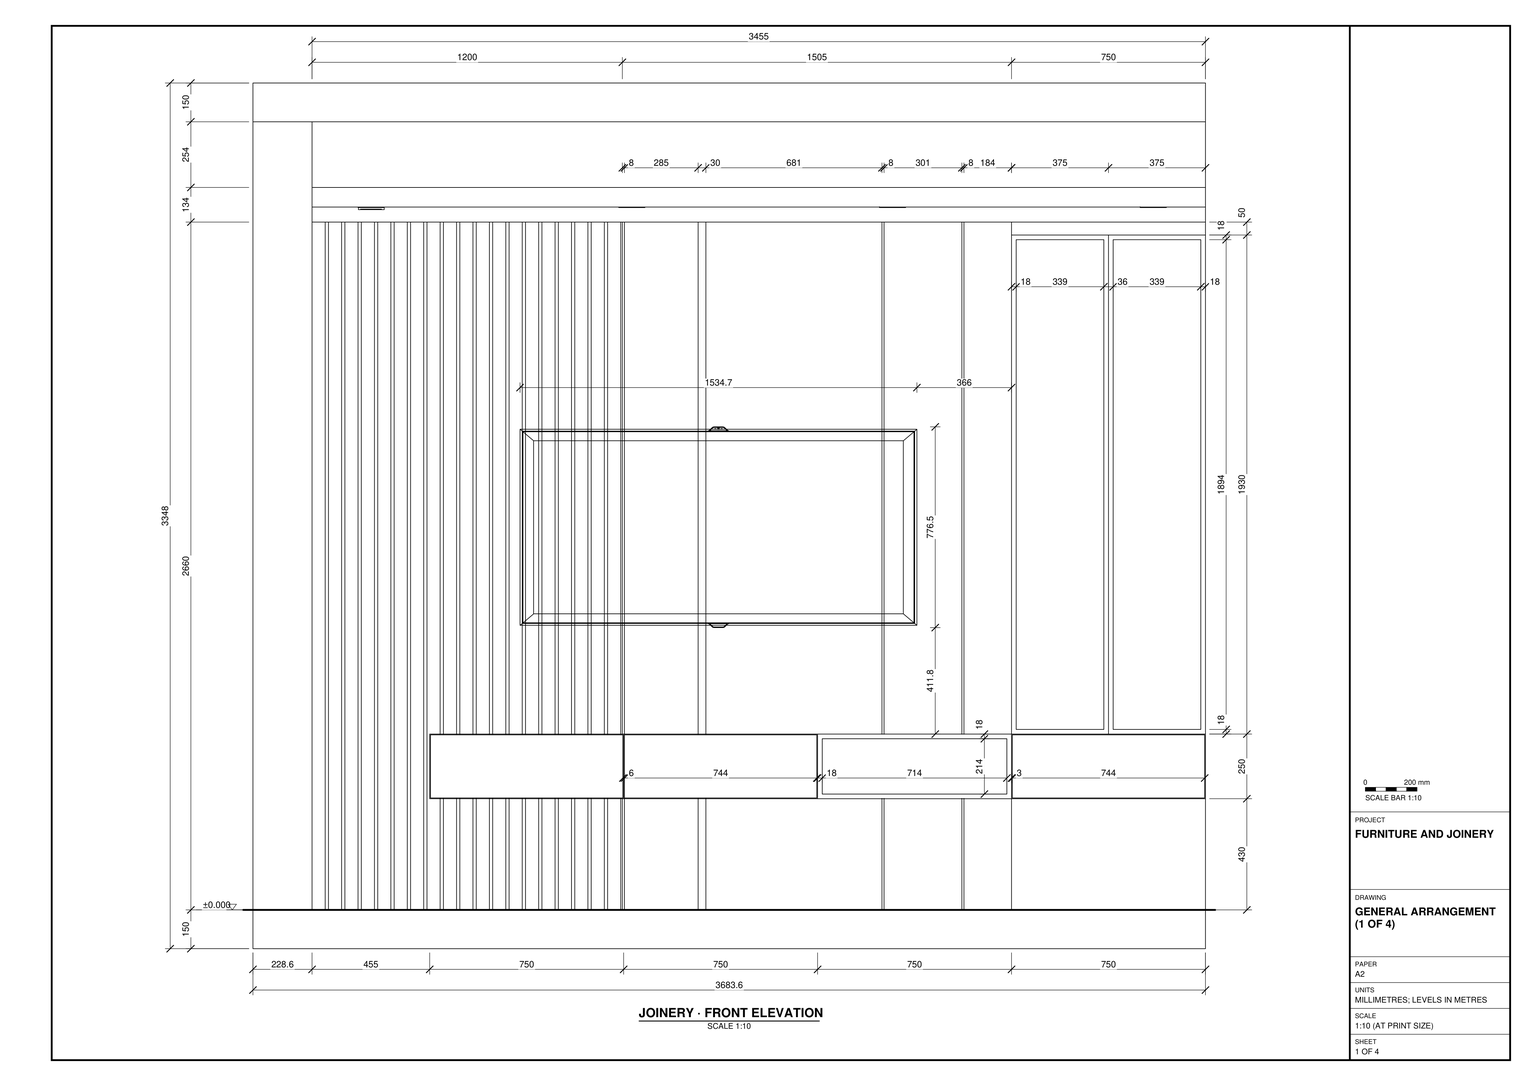
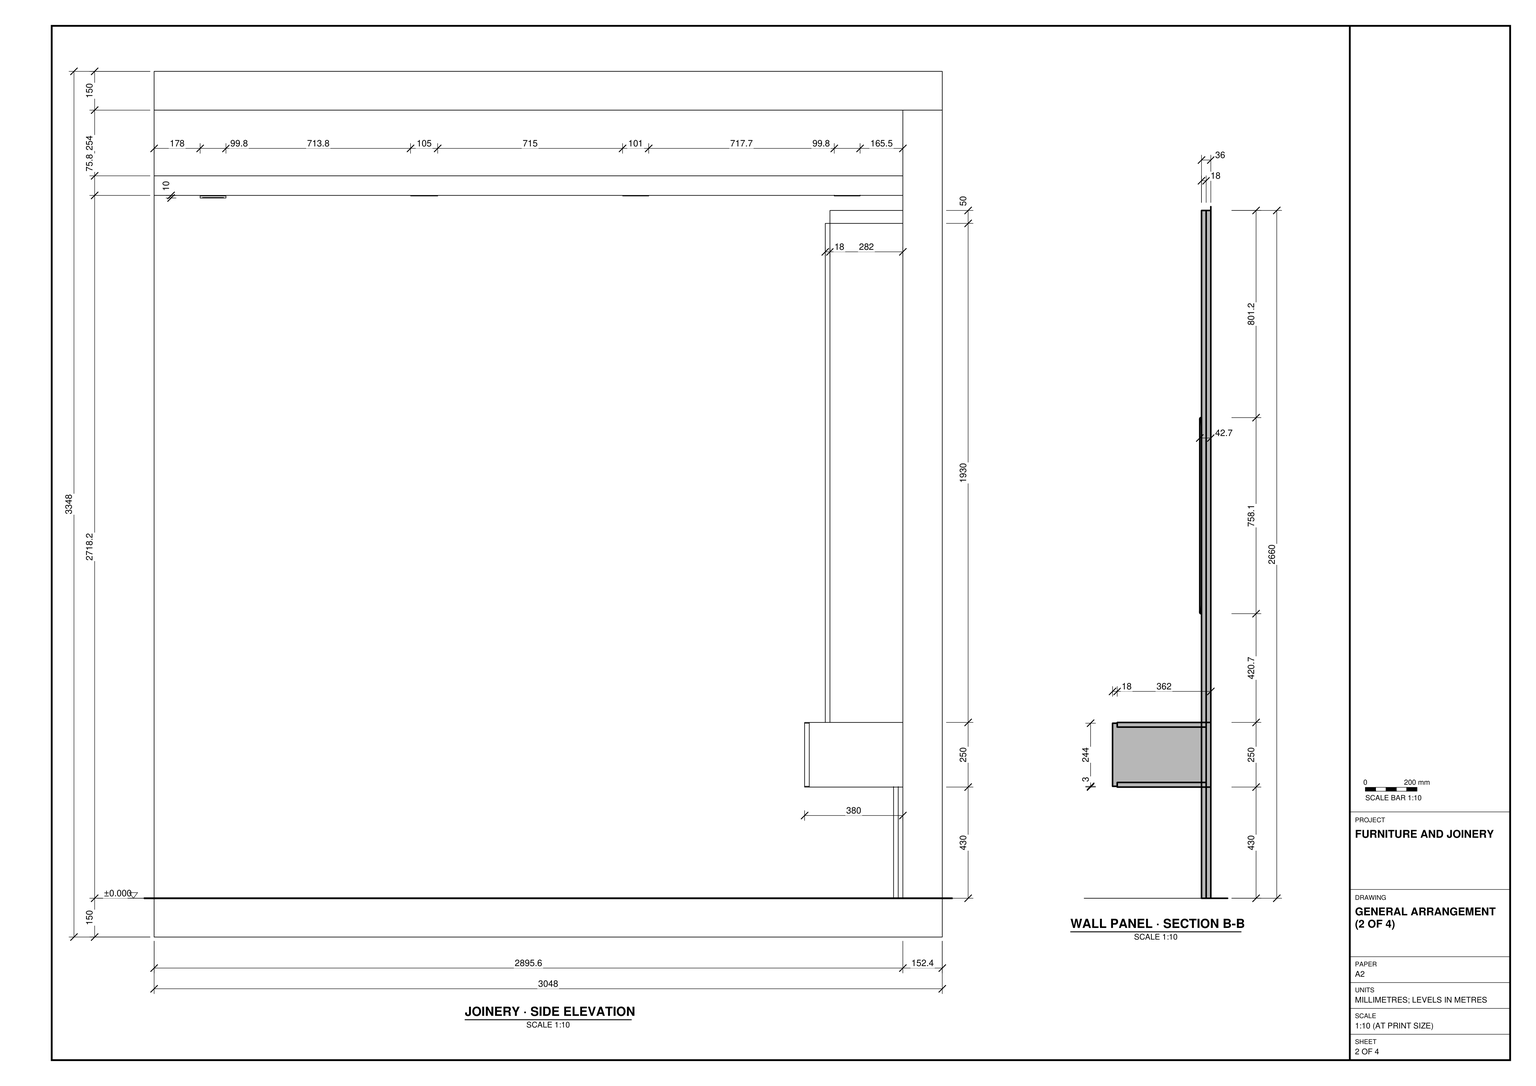
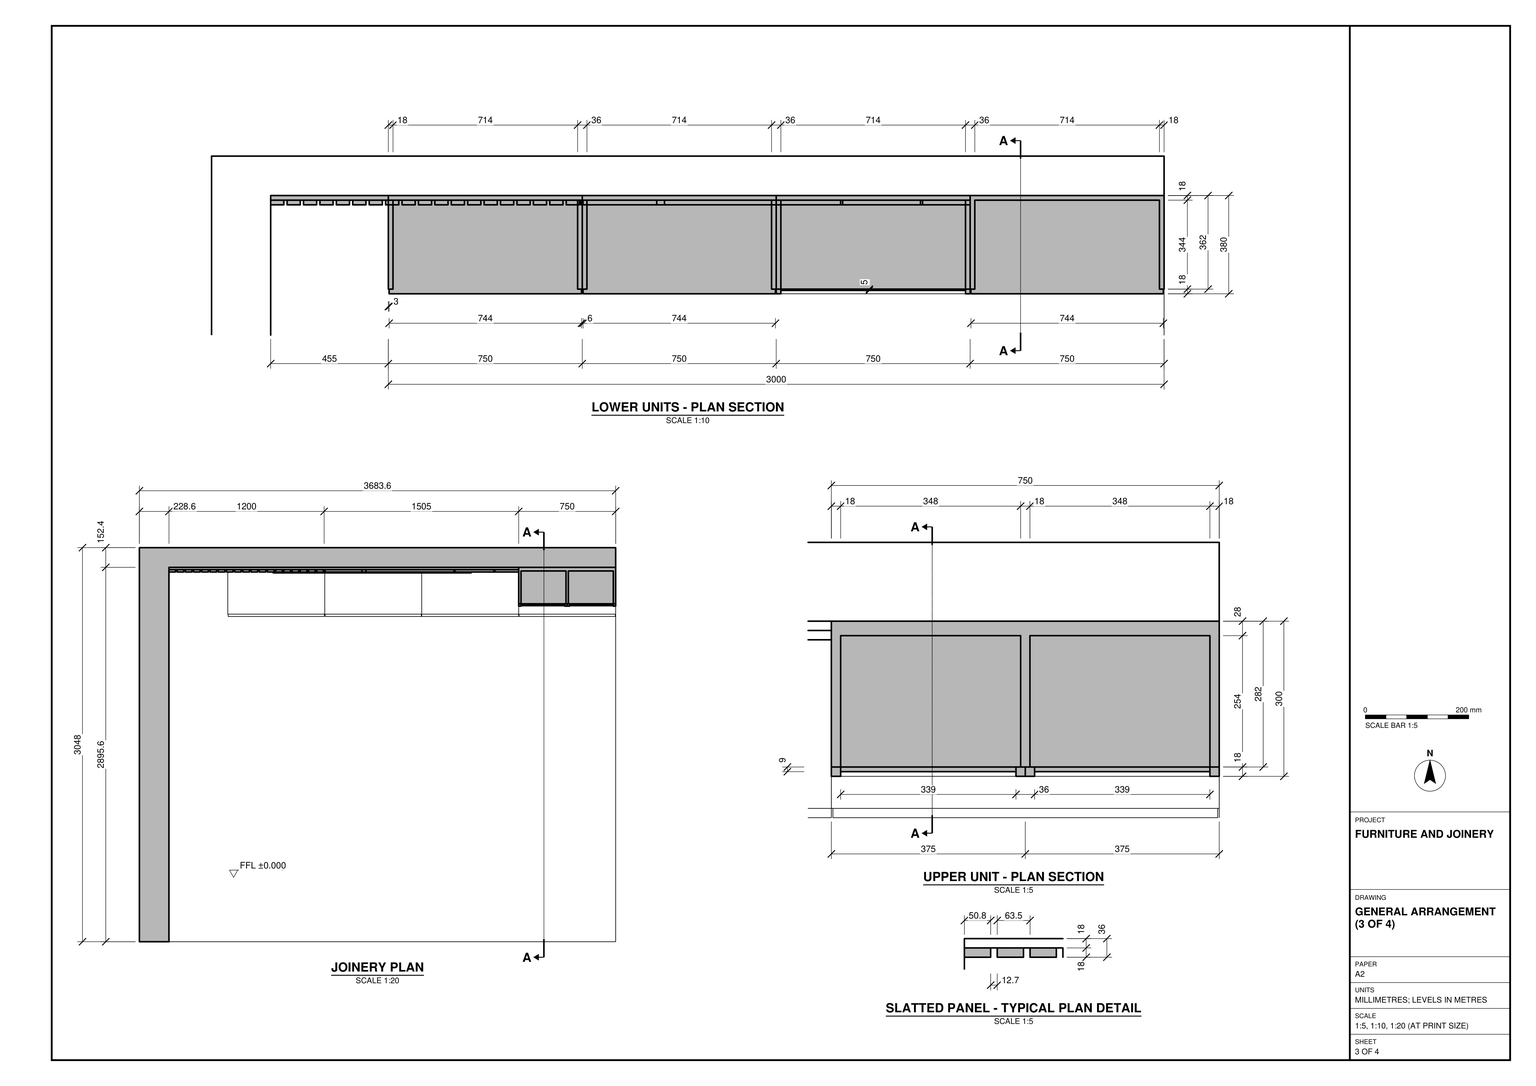
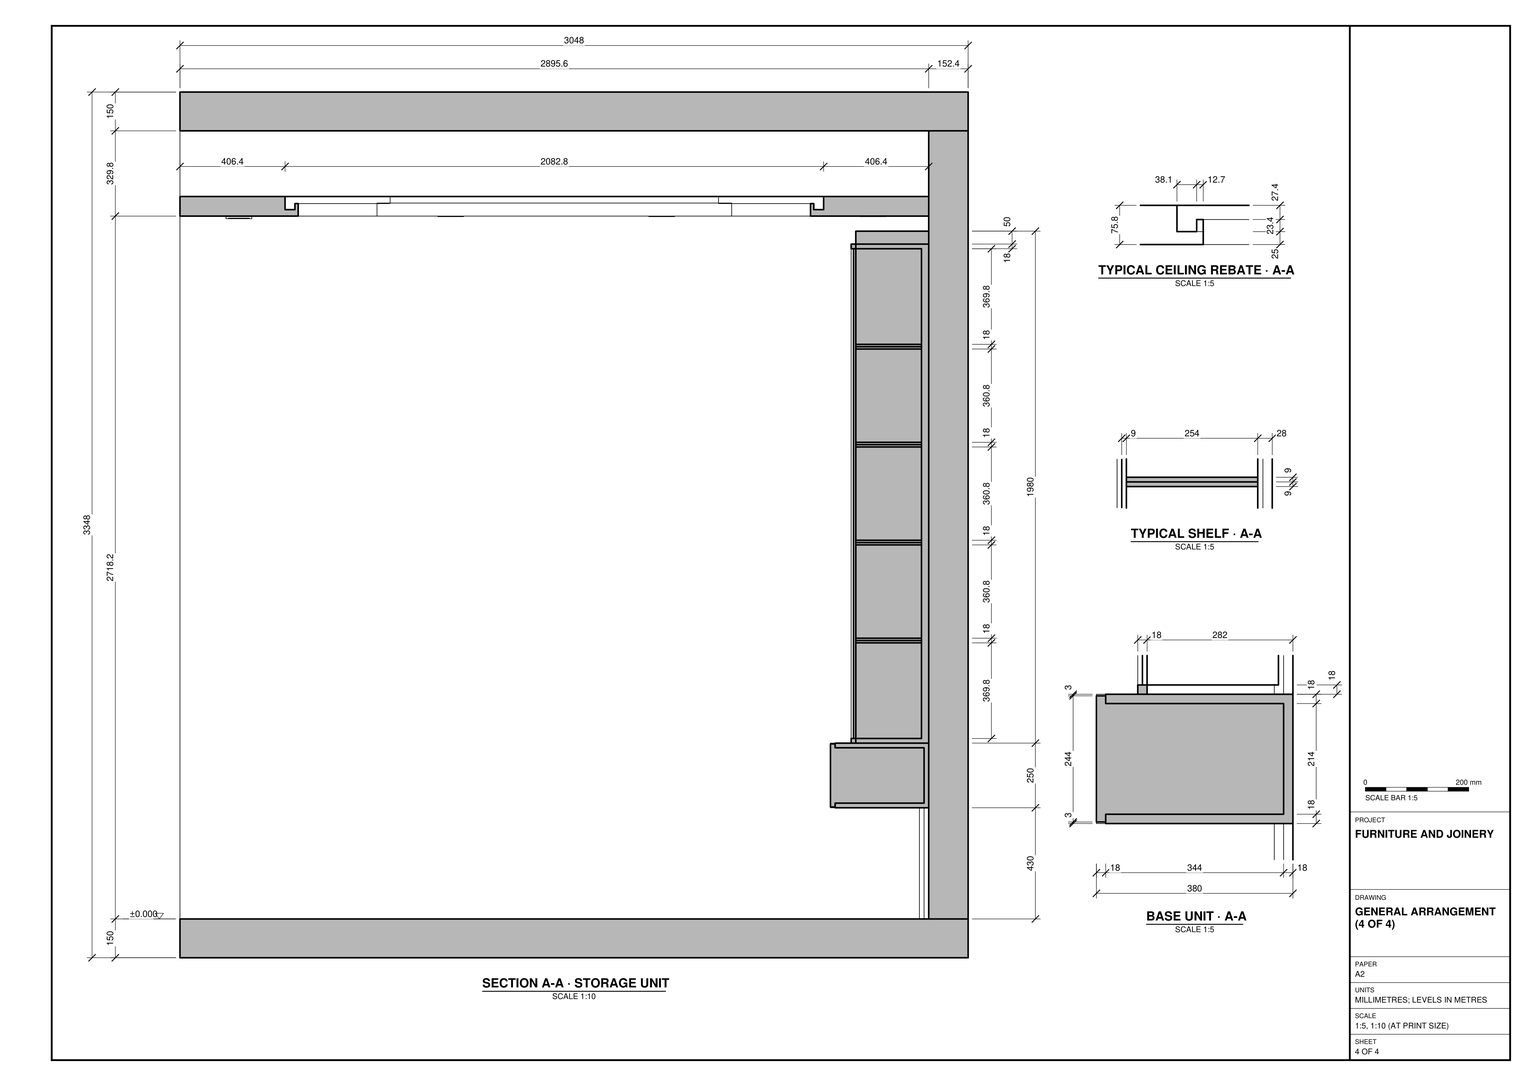
Work in millimetres in SketchUp. Use task_files/diagram_01.pdf to model the television wall and the room corner that supports it. The overall model is 3683.6 mm wide, 3048 mm deep and 3348 mm high, with the finished floor at 0 mm. Build the floor and overhead slabs, the 152.4 mm thick back wall and the 228.6 mm thick left return wall. Follow the elevations for the stepped soffit above the joinery.

Set out the back wall from left to right: a 1200 mm wide field of vertical slats, 1505 mm of flat panelling with the panel joints as drawn, and a 750 mm wide upper cabinet. Use the slat plan detail to model the individual slats and their backing. Mount the television across the junction between the slats and the flat panels. Below it, model the floating lower units as a continuous run of four equal bays. Leave the third bay from the left open, and align the shallower, twin-fronted upper cabinet with the rightmost bay. Use the plan sections for the cabinet depths, partitions and front clearances.

Keep shell elements and individual furniture or joinery pieces in separate groups or components, and use components for repeated parts. Decor and loose items may be represented by any suitable library component. Save one SketchUp model as output_files/slatted_television_wall_with_floating_cabinets.skp.

# SketchUp Ruby script. Lengths in millimetres.
U = 1.mm
M = Sketchup.active_model
def pt(a) = Geom::Point3d.new(a.map { |v| v * U })
def face(e, loops, mat)
  f = e.add_face(loops[0].map { |a| pt(a) })
  loops[1..].each { |l| e.add_face(l.map { |a| pt(a) }).erase! }
  f.material = f.back_material = mat if mat
  f
end
# faces: each face lists its corners as indices into pts; further lists are holes
def faces(e, pts, list, mat = nil) = list.each { |f| face(e, (f[0].is_a?(Array) ? f : [f]).map { |l| l.map { |i| pts[i] } }, mat) }
# xy, xz, yz: faces in a plane at the given z, y or x. An outline is a flat list of corners, or four numbers for a rectangle; further outlines are holes
def ring(l) = l.size == 4 ? [[l[0], l[1]], [l[2], l[1]], [l[2], l[3]], [l[0], l[3]]] : l.each_slice(2).to_a
def flat(e, list, mat, &to3) = list.each { |f| face(e, (f[0].is_a?(Array) ? f : [f]).map { |l| ring(l).map { |u, v| to3.(u, v) } }, mat) }
def xy(e, z, list, mat = nil) = flat(e, list, mat) { |x, y| [x, y, z] }
def xz(e, y, list, mat = nil) = flat(e, list, mat) { |x, z| [x, y, z] }
def yz(e, x, list, mat = nil) = flat(e, list, mat) { |y, z| [x, y, z] }
def lines(e, pts, list) = list.each { |a, b| e.add_line(pt(pts[a]), pt(pts[b])) }
# prism: a flat outline (further loops are holes) pulled along v
def prism(e, loops, v, mat = nil)
  f = face(e, loops, mat); d = Geom::Vector3d.new(v.map { |x| x * U })
  f.pushpull(f.normal.samedirection?(d) ? d.length : -d.length)
end
def box(e, o, s, mat = nil) = prism(e, [[o, [o[0] + s[0], o[1], o[2]], [o[0] + s[0], o[1] + s[1], o[2]], [o[0], o[1] + s[1], o[2]]]], [0, 0, s[2]], mat)
def at(x, y, z, deg = 0) = Geom::Transformation.translation(pt([x, y, z])) * Geom::Transformation.rotation(ORIGIN, Z_AXIS, deg.degrees)
def axes(o, x, y, z) = Geom::Transformation.new([*x, 0, *y, 0, *z, 0, *pt(o).to_a, 1])
def part(name) = M.definitions.add(name)
# library, detail: a bought-in or finely detailed component or shape, given as its bounding box
def library(name, o, s) = part(name).tap { |d| box(d.entities, o, s) }
def detail(e, o, s) = box(e.add_group.entities, o, s)
def put(e, d, t, mat = nil) = e.add_instance(d, t).tap { |i| i.material = mat if mat }
def group(e, t, mat = nil) = e.add_group.tap { |g| g.transformation = t; g.material = mat if mat }.entities
root = M.entities
M.materials.add("0209 AP 9428 SKY PINK").color = [239, 232, 229]
M.materials.add("0235 AP 9121 dancing pink").color = [200, 173, 206]
M.materials.add("[0128_White]").color = [255, 255, 255]
M.materials.add("[0130_Gainsboro]").color = [220, 220, 220]
M.materials.add("[0137_Black]").color = [0, 0, 0]
M.materials.add("[Translucent Glass Blue]").color = [100, 149, 237]
M.materials.add("[Wood Cherry Original]").color = [152, 86, 42]
M.materials.add("[Wood Veneer 01]").color = [120, 70, 37]
c1 = library("Television screen",[0,35.9,29],[912.5,6.9,513.2])
c2 = part("WOODEN PANELLING")
box(c2.entities,[0,-18,-2660],[50.8,18,2660],"[Wood Veneer 01]")
c3 = part("Group\#12")
xy(c3.entities,0,[[0,0,750,362]])
xy(c3.entities,18,[[18,0,732,344]])
xy(c3.entities,232,[[18,0,732,344]])
xy(c3.entities,250,[[0,0,750,362]])
xz(c3.entities,0,[[[0,0,750,250],[18,18,732,232]]])
xz(c3.entities,344,[[18,18,732,232]])
xz(c3.entities,362,[[0,0,750,250]])
yz(c3.entities,0,[[0,0,362,250]])
yz(c3.entities,18,[[0,18,344,232]])
yz(c3.entities,732,[[0,18,344,232]])
yz(c3.entities,750,[[0,0,362,250]])
c4 = part("Group\#4")
xy(c4.entities,3,[[3,0,747,18]])
xy(c4.entities,247,[[3,0,747,18]])
xz(c4.entities,0,[[3,3,747,247]])
xz(c4.entities,18,[[[0,0,750,250],[3,3,747,247]]])
yz(c4.entities,3,[[0,3,18,247]])
yz(c4.entities,747,[[0,3,18,247]])
c5 = part("Group\#21")
box(c5.entities,[-2669.7,0,0],[3683.6,3048,150])
c6 = library("Difference",[0,0,-331.8],[3455,2895.6,77.8])
put(root,c1,axes([1032.9,2816.8,1047.9],[1.6819,0,0],[0,1,0],[0,0,1.51307]))
g1 = group(root,at(0,2438.4,0),"0235 AP 9121 dancing pink")
prism(g1,[[[0,609.6,0],[3683.6,609.6,0],[3683.6,457.2,0],[228.6,457.2,0],[228.6,-2438.4,0],[0,-2438.4,0]]],[0,0,3048],"0209 AP 9428 SKY PINK")
g2 = group(root,at(228.6,2877.6,0))
box(g2,[0,0,0],[2705,18,2660])
put(g2,c2,at(0,0,2660))
put(g2,c2,at(63.5,0,2660))
put(g2,c2,at(127,0,2660))
put(g2,c2,at(190.5,0,2660))
put(g2,c2,at(254,0,2660))
put(g2,c2,at(317.5,0,2660))
put(g2,c2,at(381,0,2660))
put(g2,c2,at(444.5,0,2660))
put(g2,c2,at(508,0,2660))
put(g2,c2,at(571.5,0,2660))
put(g2,c2,at(635,0,2660))
put(g2,c2,at(698.5,0,2660))
put(g2,c2,at(762,0,2660))
put(g2,c2,at(825.5,0,2660))
put(g2,c2,at(889,0,2660))
put(g2,c2,at(952.5,0,2660))
put(g2,c2,at(1016,0,2660))
put(g2,c2,at(1079.5,0,2660))
put(g2,c2,at(1143,0,2660))
g3 = group(root,at(228.6,2859.6,0))
xy(g3,0,[[1200,0,1208,18],[1208,0,1493,18],[1493,0,1523,18],[1523,0,2204,18],[2204,0,2212,18],
  [2212,0,2513,18],[2513,0,2521,18],[2521,0,2705,18]])
xy(g3,2660,[[1200,0,1208,18],[1208,0,1493,18],[1493,0,1523,18],[1523,0,2204,18],[2204,0,2212,18],
  [2212,0,2513,18],[2513,0,2521,18],[2521,0,2705,18]])
xz(g3,0,[[1200,0,1208,2660],[1208,0,1493,2660],[1493,0,1523,2660],[1523,0,2204,2660],[2204,0,2212,2660],
  [2212,0,2513,2660],[2513,0,2521,2660],[2521,0,2705,2660]])
xz(g3,18,[[1208,0,1493,2660],[1493,0,1523,2660],[1523,0,2204,2660],[2204,0,2212,2660],[2212,0,2513,2660],
  [2513,0,2521,2660],[2521,0,2705,2660]])
yz(g3,1200,[[0,0,18,2660]])
yz(g3,1208,[[0,0,18,2660]])
yz(g3,1493,[[0,0,18,2660]])
yz(g3,1523,[[0,0,18,2660]])
yz(g3,2204,[[0,0,18,2660]])
yz(g3,2212,[[0,0,18,2660]])
yz(g3,2513,[[0,0,18,2660]])
yz(g3,2521,[[0,0,18,2660]])
yz(g3,2705,[[0,0,18,2660]])
put(root,c3,at(683.6,2533.6,430),"[Wood Veneer 01]")
put(root,c4,at(683.6,2515.6,430),"[Wood Cherry Original]")
g4 = group(root,at(1433.6,2533.6,430),"[Wood Veneer 01]")
xy(g4,0,[[0,0,750,362]])
xy(g4,18,[[18,0,732,344]])
xy(g4,232,[[18,0,732,344]])
xy(g4,250,[[0,0,750,362]])
xz(g4,0,[[[0,0,750,250],[18,18,732,232]]])
xz(g4,344,[[18,18,732,232]])
xz(g4,362,[[0,0,750,250]])
yz(g4,0,[[0,0,362,250]])
yz(g4,18,[[0,18,344,232]])
yz(g4,732,[[0,18,344,232]])
yz(g4,750,[[0,0,362,250]])
put(root,c4,at(1433.6,2515.6,430),"[Wood Cherry Original]")
put(root,c3,at(2183.6,2533.6,430),"[Wood Veneer 01]")
put(root,c3,at(2933.6,2533.6,430),"[Wood Veneer 01]")
put(root,c4,at(2933.6,2515.6,430),"[Wood Cherry Original]")
g5 = group(root,at(2183.6,2533.6,430),"[0137_Black]")
prism(g5,[[[0,0,0],[0,0,250],[750,0,250],[750,0,0]],[[18,0,18],[732,0,18],[732,0,232],[18,0,232]]],[0,-18,0])
g6 = group(root,at(2201.6,2533.6,448),"[Translucent Glass Blue]")
box(g6,[0,-5,0],[714,5,214])
g7 = group(root,at(2933.6,2613.6,680),"[Wood Cherry Original]")
xy(g7,0,[[0,0,750,282]])
xy(g7,18,[[18,0,366,254],[384,0,732,254]])
xy(g7,387.8,[[18,0,366,254],[384,0,732,254]])
xy(g7,396.8,[[18,0,366,254],[384,0,732,254]])
xy(g7,405.8,[[18,0,366,254],[384,0,732,254]])
xy(g7,766.6,[[18,0,366,254],[384,0,732,254]])
xy(g7,775.6,[[18,0,366,254],[384,0,732,254]])
xy(g7,784.6,[[18,0,366,254],[384,0,732,254]])
xy(g7,1145.4,[[18,0,366,254],[384,0,732,254]])
xy(g7,1154.4,[[18,0,366,254],[384,0,732,254]])
xy(g7,1163.4,[[18,0,366,254],[384,0,732,254]])
xy(g7,1524.2,[[18,0,366,254],[384,0,732,254]])
xy(g7,1533.2,[[18,0,366,254],[384,0,732,254]])
xy(g7,1542.2,[[18,0,366,254],[384,0,732,254]])
xy(g7,1912,[[18,0,366,254],[384,0,732,254]])
xy(g7,1930,[[0,0,750,282]])
xy(g7,1980,[[0,0,750,282]])
xz(g7,0,[[[0,0,750,1930],[18,18,732,1912]],[366,18,384,1912],[18,387.8,366,396.8],[384,387.8,732,396.8],[18,396.8,366,405.8],
  [384,396.8,732,405.8],[18,766.6,366,775.6],[384,766.6,732,775.6],[18,775.6,366,784.6],[384,775.6,732,784.6],
  [18,1145.4,366,1154.4],[384,1145.4,732,1154.4],[18,1154.4,366,1163.4],[384,1154.4,732,1163.4],[18,1524.2,366,1533.2],
  [384,1524.2,732,1533.2],[18,1533.2,366,1542.2],[384,1533.2,732,1542.2],[0,1930,750,1980]])
xz(g7,254,[[18,18,366,387.8],[384,18,732,387.8],[18,387.8,366,396.8],[384,387.8,732,396.8],[18,396.8,366,405.8],
  [384,396.8,732,405.8],[18,405.8,366,766.6],[384,405.8,732,766.6],[18,766.6,366,775.6],[384,766.6,732,775.6],
  [18,775.6,366,784.6],[384,775.6,732,784.6],[18,784.6,366,1145.4],[384,784.6,732,1145.4],[18,1145.4,366,1154.4],
  [384,1145.4,732,1154.4],[18,1154.4,366,1163.4],[384,1154.4,732,1163.4],[18,1163.4,366,1524.2],[384,1163.4,732,1524.2],
  [18,1524.2,366,1533.2],[384,1524.2,732,1533.2],[18,1533.2,366,1542.2],[384,1533.2,732,1542.2],[18,1542.2,366,1912],
  [384,1542.2,732,1912]])
xz(g7,282,[[0,0,750,1930],[0,1930,750,1980]])
yz(g7,0,[[0,0,282,1930],[0,1930,282,1980]])
yz(g7,18,[[0,18,254,387.8],[0,387.8,254,396.8],[0,396.8,254,405.8],[0,405.8,254,766.6],[0,766.6,254,775.6],
  [0,775.6,254,784.6],[0,784.6,254,1145.4],[0,1145.4,254,1154.4],[0,1154.4,254,1163.4],[0,1163.4,254,1524.2],
  [0,1524.2,254,1533.2],[0,1533.2,254,1542.2],[0,1542.2,254,1912]])
yz(g7,366,[[0,18,254,387.8],[0,387.8,254,396.8],[0,396.8,254,405.8],[0,405.8,254,766.6],[0,766.6,254,775.6],
  [0,775.6,254,784.6],[0,784.6,254,1145.4],[0,1145.4,254,1154.4],[0,1154.4,254,1163.4],[0,1163.4,254,1524.2],
  [0,1524.2,254,1533.2],[0,1533.2,254,1542.2],[0,1542.2,254,1912]])
yz(g7,384,[[0,18,254,387.8],[0,387.8,254,396.8],[0,396.8,254,405.8],[0,405.8,254,766.6],[0,766.6,254,775.6],
  [0,775.6,254,784.6],[0,784.6,254,1145.4],[0,1145.4,254,1154.4],[0,1154.4,254,1163.4],[0,1163.4,254,1524.2],
  [0,1524.2,254,1533.2],[0,1533.2,254,1542.2],[0,1542.2,254,1912]])
yz(g7,732,[[0,18,254,387.8],[0,387.8,254,396.8],[0,396.8,254,405.8],[0,405.8,254,766.6],[0,766.6,254,775.6],
  [0,775.6,254,784.6],[0,784.6,254,1145.4],[0,1145.4,254,1154.4],[0,1154.4,254,1163.4],[0,1163.4,254,1524.2],
  [0,1524.2,254,1533.2],[0,1533.2,254,1542.2],[0,1542.2,254,1912]])
yz(g7,750,[[0,0,282,1930],[0,1930,282,1980]])
g8 = group(root,at(2933.6,2595.6,680),"[0137_Black]")
prism(g8,[[[0,18,0],[0,18,1930],[375,18,1930],[375,18,0]],[[18,18,18],[357,18,18],[357,18,1912],[18,18,1912]]],[0,-18,0])
g9 = group(root,at(2951.6,2613.6,698),"[Translucent Glass Blue]")
box(g9,[0,-9,0],[339,9,1894])
g10 = group(root,at(3308.6,2595.6,680),"[0137_Black]")
prism(g10,[[[375,18,1930],[375,18,0],[0,18,0],[0,18,1930]],[[18,18,18],[357,18,18],[357,18,1912],[18,18,1912]]],[0,-18,0])
g11 = group(root,at(3326.6,2613.6,698),"[Translucent Glass Blue]")
box(g11,[0,-9,0],[339,9,1894])
put(root,c5,at(2669.7,0,-150))
put(root,c6,at(228.6,0,3048))
g12 = group(root,at(407.8,178,2708.2))
xy(g12,0,[[[46.9,0,40.6,0.8,34.5,2.3,28.7,4.7,23.2,7.7,18.1,11.4,13.6,15.7,9.5,20.5,6.2,25.8,3.5,31.5,1.6,37.5,0.4,43.6,0,49.9,0.4,56.2,1.6,62.3,3.5,68.3,6.2,74,9.5,79.3,13.6,84.1,18.1,88.4,23.2,92.1,28.7,95.1,34.5,97.5,40.6,99,46.9,99.8,53.1,99.8,59.4,99,65.5,97.5,71.3,95.1,76.8,92.1,81.9,88.4,86.4,84.1,90.5,79.3,93.8,74,96.5,68.3,98.4,62.3,99.6,56.2,100,49.9,99.6,43.6,98.4,37.5,96.5,31.5,93.8,25.8,90.5,20.5,86.4,15.7,81.9,11.4,76.8,7.7,71.3,4.7,65.5,2.3,59.4,0.8,53.1,0],[47.2,5,52.8,5,58.4,5.7,63.9,7.1,69.2,9.2,74.1,11.9,78.7,15.2,82.8,19.1,86.4,23.5,89.4,28.2,91.8,33.3,93.6,38.7,94.6,44.3,95,49.9,94.6,55.5,93.6,61.1,91.8,66.5,89.4,71.6,86.4,76.4,82.8,80.7,78.7,84.6,74.1,87.9,69.2,90.6,63.9,92.7,58.4,94.1,52.8,94.8,47.2,94.8,41.6,94.1,36.1,92.7,30.8,90.6,25.9,87.9,21.3,84.6,17.2,80.7,13.6,76.4,10.6,71.6,8.2,66.5,6.4,61.1,5.4,55.5,5,49.9,5.4,44.3,6.4,38.7,8.2,33.3,10.6,28.2,13.6,23.5,17.2,19.1,21.3,15.2,25.9,11.9,30.8,9.2,36.1,7.1,41.6,5.7]]],"[0130_Gainsboro]")
xy(g12,2,[[47.2,5,41.6,5.7,36.1,7.1,30.8,9.2,25.9,11.9,21.3,15.2,17.2,19.1,13.6,23.5,10.6,28.2,8.2,33.3,6.4,38.7,5.4,44.3,5,49.9,5.4,55.5,6.4,61.1,8.2,66.5,10.6,71.6,13.6,76.4,17.2,80.7,21.3,84.6,25.9,87.9,30.8,90.6,36.1,92.7,41.6,94.1,47.2,94.8,52.8,94.8,58.4,94.1,63.9,92.7,69.2,90.6,74.1,87.9,78.7,84.6,82.8,80.7,86.4,76.4,89.4,71.6,91.8,66.5,93.6,61.1,94.6,55.5,95,49.9,94.6,44.3,93.6,38.7,91.8,33.3,89.4,28.2,86.4,23.5,82.8,19.1,78.7,15.2,74.1,11.9,69.2,9.2,63.9,7.1,58.4,5.7,52.8,5]],"[0128_White]")
xy(g12,10,[[46.9,0,53.1,0,59.4,0.8,65.5,2.3,71.3,4.7,76.8,7.7,81.9,11.4,86.4,15.7,90.5,20.5,93.8,25.8,96.5,31.5,98.4,37.5,99.6,43.6,100,49.9,99.6,56.2,98.4,62.3,96.5,68.3,93.8,74,90.5,79.3,86.4,84.1,81.9,88.4,76.8,92.1,71.3,95.1,65.5,97.5,59.4,99,53.1,99.8,46.9,99.8,40.6,99,34.5,97.5,28.7,95.1,23.2,92.1,18.1,88.4,13.6,84.1,9.5,79.3,6.2,74,3.5,68.3,1.6,62.3,0.4,56.2,0,49.9,0.4,43.6,1.6,37.5,3.5,31.5,6.2,25.8,9.5,20.5,13.6,15.7,18.1,11.4,23.2,7.7,28.7,4.7,34.5,2.3,40.6,0.8]],"[0130_Gainsboro]")
xz(g12,0,[[46.9,0,53.1,10]],"[0130_Gainsboro]")
xz(g12,5,[[47.2,0,52.8,2]],"[0130_Gainsboro]")
xz(g12,94.8,[[47.2,0,52.8,2]],"[0130_Gainsboro]")
xz(g12,99.8,[[46.9,0,53.1,10]],"[0130_Gainsboro]")
p = [[40.6,0.8,0],[46.9,0,0],[46.9,0,10],[40.6,0.8,10],[53.1,0,0],[59.4,0.8,0],
  [59.4,0.8,10],[53.1,0,10],[34.5,2.3,0],[34.5,2.3,10],[65.5,2.3,0],[65.5,2.3,10],
  [28.7,4.7,0],[28.7,4.7,10],[71.3,4.7,0],[71.3,4.7,10],[23.2,7.7,0],[23.2,7.7,10],
  [76.8,7.7,0],[76.8,7.7,10],[47.2,5,0],[41.6,5.7,0],[41.6,5.7,2],[47.2,5,2],
  [58.4,5.7,0],[52.8,5,0],[52.8,5,2],[58.4,5.7,2],[36.1,7.1,0],[36.1,7.1,2],
  [63.9,7.1,0],[63.9,7.1,2],[30.8,9.2,0],[30.8,9.2,2],[69.2,9.2,0],[69.2,9.2,2],
  [18.1,11.4,0],[18.1,11.4,10],[81.9,11.4,0],[81.9,11.4,10],[25.9,11.9,0],[25.9,11.9,2],
  [74.1,11.9,0],[74.1,11.9,2],[13.6,15.7,0],[13.6,15.7,10],[86.4,15.7,0],[86.4,15.7,10],
  [21.3,15.2,0],[21.3,15.2,2],[78.7,15.2,0],[78.7,15.2,2],[17.2,19.1,0],[17.2,19.1,2],
  [82.8,19.1,0],[82.8,19.1,2],[9.5,20.5,0],[9.5,20.5,10],[90.5,20.5,0],[90.5,20.5,10],
  [13.6,23.5,0],[13.6,23.5,2],[86.4,23.5,0],[86.4,23.5,2],[6.2,25.8,0],[6.2,25.8,10],
  [93.8,25.8,0],[93.8,25.8,10],[10.6,28.2,0],[10.6,28.2,2],[89.4,28.2,0],[89.4,28.2,2],
  [3.5,31.5,0],[3.5,31.5,10],[96.5,31.5,0],[96.5,31.5,10],[8.2,33.3,0],[8.2,33.3,2],
  [91.8,33.3,0],[91.8,33.3,2],[1.6,37.5,0],[1.6,37.5,10],[98.4,37.5,0],[98.4,37.5,10],
  [6.4,38.7,0],[6.4,38.7,2],[93.6,38.7,0],[93.6,38.7,2],[0.4,43.6,0],[0.4,43.6,10],
  [99.6,43.6,0],[99.6,43.6,10],[5.4,44.3,0],[5.4,44.3,2],[94.6,44.3,0],[94.6,44.3,2],
  [0,49.9,0],[0,49.9,10],[100,49.9,0],[100,49.9,10],[5,49.9,0],[5,49.9,2],
  [95,49.9,0],[95,49.9,2],[0.4,56.2,0],[0.4,56.2,10],[5.4,55.5,0],[5.4,55.5,2],
  [94.6,55.5,0],[94.6,55.5,2],[99.6,56.2,0],[99.6,56.2,10],[6.4,61.1,0],[6.4,61.1,2],
  [93.6,61.1,0],[93.6,61.1,2],[1.6,62.3,0],[1.6,62.3,10],[98.4,62.3,0],[98.4,62.3,10],
  [8.2,66.5,0],[8.2,66.5,2],[91.8,66.5,0],[91.8,66.5,2],[3.5,68.3,0],[3.5,68.3,10],
  [96.5,68.3,0],[96.5,68.3,10],[10.6,71.6,0],[10.6,71.6,2],[89.4,71.6,0],[89.4,71.6,2],
  [6.2,74,0],[6.2,74,10],[93.8,74,0],[93.8,74,10],[13.6,76.4,0],[13.6,76.4,2],
  [86.4,76.4,0],[86.4,76.4,2],[9.5,79.3,0],[9.5,79.3,10],[90.5,79.3,0],[90.5,79.3,10],
  [17.2,80.7,0],[17.2,80.7,2],[82.8,80.7,0],[82.8,80.7,2],[13.6,84.1,0],[13.6,84.1,10],
  [86.4,84.1,0],[86.4,84.1,10],[21.3,84.6,0],[21.3,84.6,2],[78.7,84.6,0],[78.7,84.6,2],
  [18.1,88.4,0],[18.1,88.4,10],[81.9,88.4,0],[81.9,88.4,10],[25.9,87.9,0],[25.9,87.9,2],
  [74.1,87.9,0],[74.1,87.9,2],[30.8,90.6,0],[30.8,90.6,2],[69.2,90.6,0],[69.2,90.6,2],
  [23.2,92.1,0],[23.2,92.1,10],[76.8,92.1,0],[76.8,92.1,10],[36.1,92.7,0],[36.1,92.7,2],
  [63.9,92.7,0],[63.9,92.7,2],[28.7,95.1,0],[28.7,95.1,10],[71.3,95.1,0],[71.3,95.1,10],
  [41.6,94.1,0],[41.6,94.1,2],[58.4,94.1,0],[58.4,94.1,2],[47.2,94.8,0],[47.2,94.8,2],
  [52.8,94.8,0],[52.8,94.8,2],[34.5,97.5,0],[34.5,97.5,10],[65.5,97.5,0],[65.5,97.5,10],
  [40.6,99,0],[40.6,99,10],[59.4,99,0],[59.4,99,10],[46.9,99.8,0],[46.9,99.8,10],
  [53.1,99.8,0],[53.1,99.8,10]]
faces(g12,p,[[0,1,2,3],[4,5,6,7],[8,0,3,9],[5,10,11,6],[12,8,9,13],[10,14,15,11],[16,12,13,17],[14,18,19,15],
  [20,21,22,23],[24,25,26,27],[21,28,29,22],[30,24,27,31],[28,32,33,29],[34,30,31,35],[36,16,17,37],[18,38,39,19],
  [32,40,41,33],[42,34,35,43],[44,36,37,45],[38,46,47,39],[40,48,49,41],[50,42,43,51],[48,52,53,49],[54,50,51,55],
  [56,44,45,57],[46,58,59,47],[52,60,61,53],[62,54,55,63],[64,56,57,65],[58,66,67,59],[60,68,69,61],[70,62,63,71],
  [72,64,65,73],[66,74,75,67],[68,76,77,69],[78,70,71,79],[80,72,73,81],[74,82,83,75],[76,84,85,77],[86,78,79,87],
  [88,80,81,89],[82,90,91,83],[84,92,93,85],[94,86,87,95],[96,88,89,97],[90,98,99,91],[92,100,101,93],[102,94,95,103],
  [104,96,97,105],[100,106,107,101],[108,102,103,109],[98,110,111,99],[106,112,113,107],[114,108,109,115],[116,104,105,117],[110,118,119,111],
  [112,120,121,113],[122,114,115,123],[124,116,117,125],[118,126,127,119],[120,128,129,121],[130,122,123,131],[132,124,125,133],[126,134,135,127],
  [128,136,137,129],[138,130,131,139],[140,132,133,141],[134,142,143,135],[136,144,145,137],[146,138,139,147],[148,140,141,149],[142,150,151,143],
  [144,152,153,145],[154,146,147,155],[156,148,149,157],[150,158,159,151],[152,160,161,153],[162,154,155,163],[160,164,165,161],[166,162,163,167],
  [168,156,157,169],[158,170,171,159],[164,172,173,165],[174,166,167,175],[176,168,169,177],[170,178,179,171],[172,180,181,173],[182,174,175,183],
  [180,184,185,181],[186,182,183,187],[188,176,177,189],[178,190,191,179],[192,188,189,193],[190,194,195,191],[196,192,193,197],[194,198,199,195]],"[0130_Gainsboro]")
put(root,c5,at(2669.7,0,3048))
